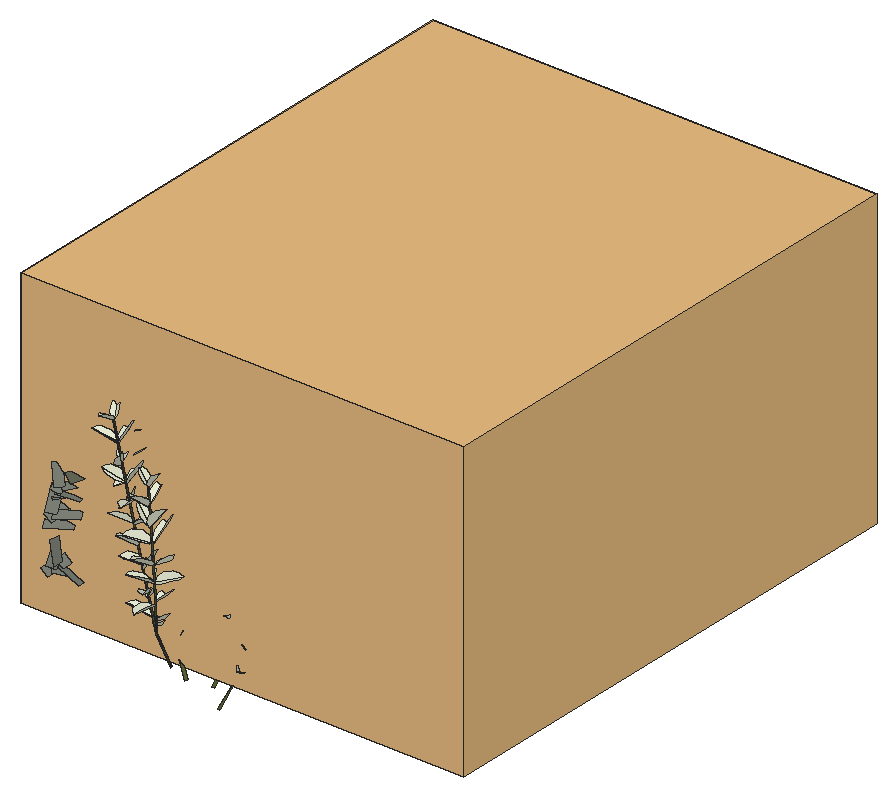
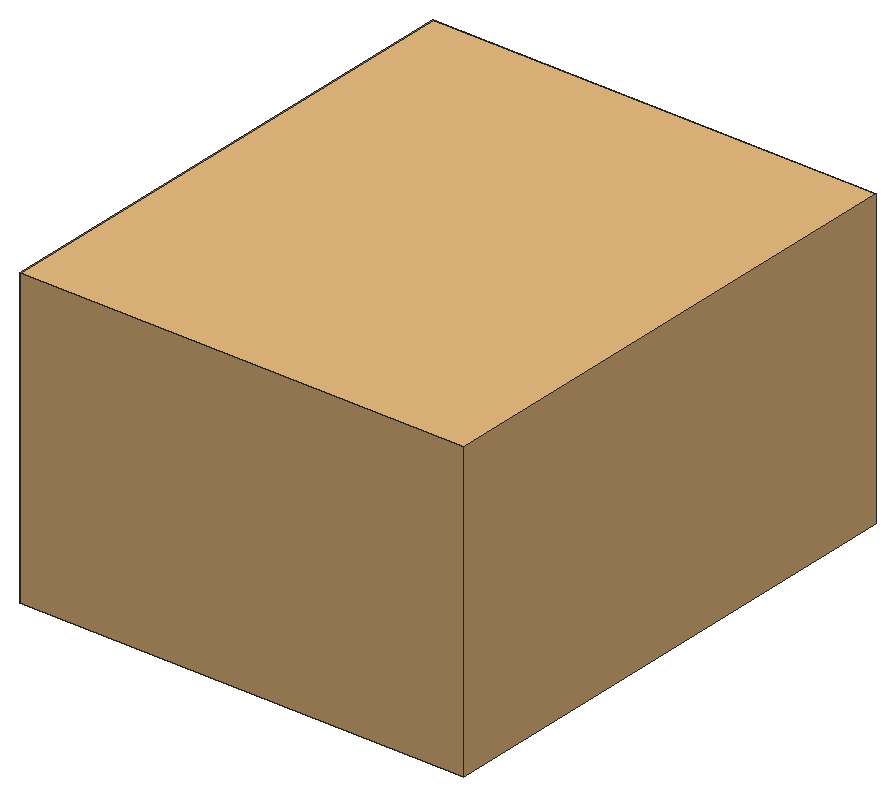
# SketchUp Ruby script. Lengths in inches.
U = 1.inch
M = Sketchup.active_model
def pt(a) = Geom::Point3d.new(a.map { |v| v * U })
def face(e, loops, mat)
  f = e.add_face(loops[0].map { |a| pt(a) })
  loops[1..].each { |l| e.add_face(l.map { |a| pt(a) }).erase! }
  f.material = f.back_material = mat if mat
  f
end
# faces: each face lists its corners as indices into pts; further lists are holes
def faces(e, pts, list, mat = nil) = list.each { |f| face(e, (f[0].is_a?(Array) ? f : [f]).map { |l| l.map { |i| pts[i] } }, mat) }
# xy, xz, yz: faces in a plane at the given z, y or x. An outline is a flat list of corners, or four numbers for a rectangle; further outlines are holes
def ring(l) = l.size == 4 ? [[l[0], l[1]], [l[2], l[1]], [l[2], l[3]], [l[0], l[3]]] : l.each_slice(2).to_a
def flat(e, list, mat, &to3) = list.each { |f| face(e, (f[0].is_a?(Array) ? f : [f]).map { |l| ring(l).map { |u, v| to3.(u, v) } }, mat) }
def xy(e, z, list, mat = nil) = flat(e, list, mat) { |x, y| [x, y, z] }
def xz(e, y, list, mat = nil) = flat(e, list, mat) { |x, z| [x, y, z] }
def yz(e, x, list, mat = nil) = flat(e, list, mat) { |y, z| [x, y, z] }
def lines(e, pts, list) = list.each { |a, b| e.add_line(pt(pts[a]), pt(pts[b])) }
# prism: a flat outline (further loops are holes) pulled along v
def prism(e, loops, v, mat = nil)
  f = face(e, loops, mat); d = Geom::Vector3d.new(v.map { |x| x * U })
  f.pushpull(f.normal.samedirection?(d) ? d.length : -d.length)
end
def box(e, o, s, mat = nil) = prism(e, [[o, [o[0] + s[0], o[1], o[2]], [o[0] + s[0], o[1] + s[1], o[2]], [o[0], o[1] + s[1], o[2]]]], [0, 0, s[2]], mat)
def at(x, y, z, deg = 0) = Geom::Transformation.translation(pt([x, y, z])) * Geom::Transformation.rotation(ORIGIN, Z_AXIS, deg.degrees)
def axes(o, x, y, z) = Geom::Transformation.new([*x, 0, *y, 0, *z, 0, *pt(o).to_a, 1])
def part(name) = M.definitions.add(name)
# library, detail: a bought-in or finely detailed component or shape, given as its bounding box
def library(name, o, s) = part(name).tap { |d| box(d.entities, o, s) }
def detail(e, o, s) = box(e.add_group.entities, o, s)
def put(e, d, t, mat = nil) = e.add_instance(d, t).tap { |i| i.material = mat if mat }
def group(e, t, mat = nil) = e.add_group.tap { |g| g.transformation = t; g.material = mat if mat }.entities
root = M.entities
M.materials.add("0ad16as01f6asdLeafVar1sfd015as60f1as6").color = [231, 235, 211]
M.materials.add("asdfasdf0165f6asdLeafVar1sfd015as60f1as6").color = [231, 235, 211]
M.materials.add("dw_stemssadfasdfa0sdf1s01d6w1").color = [90, 97, 50]
M.materials.add("viburnumblaasdfas0df1w06d").color = [98, 102, 84]
M.materials.add("viburnumbladsadfasdfad0w122").color = [125, 129, 119]
c1 = part("vdw_leaf\#3")
p = [[0,0,0],[-2.77,1.61,2.32],[-4.3125,6.1,4.5],[-3.97,13.49,6.09],[-2.47,18.57,6.3],[-0.2,22.73,5.75],
  [2.54,19.66,6.85],[4.3,15.93,7.09],[5.03,7.6,5.43],[3.32,1.76,2.74]]
faces(c1.entities,p,[[0,1,2,3,4,5],[0,5,6,7,8,9]],"asdfasdf0165f6asdLeafVar1sfd015as60f1as6")
c2 = part("dw_brancj_2\#2")
p = [[9.7,-0.22,29.95],[0.23,-1.96,0.34],[-0.05,1.51,0.11],[9.65,1.51,29.46],[18.64,-8.75,84.43],[18.96,-6.63,84.625],
  [1.53,6.02,63.68],[1.42,8.18,63.25],[-10.58,8.77,161.17],[-10.41,9.98,160.68],[26.34,-9.37,211.72],[26.57,-8.28,211.23]]
faces(c2.entities,p,[[0,1,2],[0,2,3],[4,0,3],[4,3,5],[6,0,3],[6,3,7],[8,6,7],[8,7,9],
  [10,4,5],[10,5,11]],"dw_stemssadfasdfa0sdf1s01d6w1")
c3 = part("vdw_branch2\#3")
put(c3.entities,c1,axes([19.53,-5.9,102.42],[1.12377,-0.50004,0],[0.46097,1.03596,0.47664],[-0.19377,-0.43548,1.13389]))
put(c3.entities,c1,axes([-5.89,6.52,109.44],[-1.07209,0.83679,0],[-0.77141,-0.98832,0.52702],[0.32427,0.41545,1.25373]))
put(c3.entities,c1,axes([-0.44,8.23,75.28],[0.88709,-0.9947,0],[0.92159,0.82189,0.33087],[-0.25219,-0.22491,1.26111]))
put(c3.entities,c1,axes([24.71,-8.97,190.81],[-0.82641,0.91101,0],[-0.83983,-0.76184,0.47664],[0.35303,0.32025,1.13389]))
put(c3.entities,c1,axes([-2.29,8.24,91.35],[1.24603,-0.47303,0],[0.43826,1.15445,0.33087],[-0.11993,-0.31592,1.26111]))
put(c3.entities,c1,axes([12.26,-3.11,37.92],[-0.64625,1.02205,0.22511],[-1.04383,-0.61044,-0.22511],[-0.07533,-0.30931,1.18809]))
put(c3.entities,c1,axes([26.17,-9.17,210.27],[-0.99452,-0.10453,0],[0.09636,-0.91681,0.38752],[-0.04051,0.38539,0.92186]))
put(c3.entities,c1,axes([-6.07,9.4,125.35],[-0.90214,-0.98107,0],[0.90896,-0.83583,0.33087],[-0.24874,0.22873,1.26111]))
put(c3.entities,c1,axes([-4.13,7.29,110.58],[0.44715,-1.078,0.64369],[1.05816,0.63649,0.33087],[-0.58725,0.40856,1.09216]))
put(c3.entities,c1,axes([23.91,-8.22,171.96],[0.62307,0.85009,-0.63406],[-0.71531,0.8798,0.47664],[0.78296,0.12729,0.94004]))
put(c3.entities,c2,at(-0.09,0.18,-0.25),"dw_stemssadfasdfa0sdf1s01d6w1")
put(c3.entities,c1,axes([23.34,-9.65,156.59],[-0.31364,-1.00782,0.58216],[1.10369,-0.17062,0.29925],[-0.17137,0.6239,0.98776]))
put(c3.entities,c1,axes([15.03,-3.37,58.83],[-1.05425,-0.00194,0.58442],[-0.14303,-1.11707,-0.26172],[0.55355,-0.3046,0.99755]))
put(c3.entities,c1,axes([-11.625,9.46,160.37],[0.36812,0.92978,0],[-0.85713,0.33936,0.38752],[0.3603,-0.14265,0.92186]))
put(c3.entities,c1,axes([21.32,-8.53,138.72],[1.21379,0.19904,0],[-0.19904,1.21379,0],[0,0,1.23]))
put(c3.entities,c1,axes([22.54,-9.2,141.43],[-1.02887,0.17955,0.60182],[-0.23387,-1.13057,-0.06253],[0.56696,-0.17376,1.02111]))
put(c3.entities,c1,axes([23.9,-8.82,173.84],[-1.14567,-0.37474,0],[0.35918,-1.0981,0.04438],[-0.01409,0.04308,1.17993]))
put(c3.entities,c1,axes([-7.84,8.92,143.59],[-1.26971,0.40522,0],[-0.37543,-1.17638,0.33087],[0.10274,0.32192,1.26111]))
put(c3.entities,c1,axes([19.77,-8.01,85.98],[-0.32405,-1.14591,0.18674],[1.10278,-0.32969,-0.10948],[0.15845,0.14442,1.16117]))
put(c3.entities,c1,axes([-0.62,5.76,76.34],[-0.08879,1.17576,-0.67771],[-1.34525,-0.16582,-0.11144],[-0.17897,0.66309,1.17383]))
put(c3.entities,c1,axes([20.49,-8.22,121.07],[0.39924,-0.78471,-0.8233],[1.08735,0.33121,0.2116],[0.09035,-0.83005,0.83495]))
put(c3.entities,c1,axes([15.15,-3.72,62.9],[1.16251,0.40128,-0.0211],[-0.39924,1.16074,0.07874],[0.0456,-0.06757,1.2273]))
put(c3.entities,c1,axes([20.72,-8.08,120.26],[-0.03693,1.2277,-0.06551],[-1.22944,-0.03698,0],[-0.00197,0.06548,1.22825]))
put(c3.entities,c1,axes([22.58,-8.36,155.57],[-0.56247,1.09386,0],[-1.00839,-0.51852,0.47664],[0.42389,0.21796,1.13389]))
put(c3.entities,c1,axes([3.97,3.13,57.96],[-1.09459,0.76041,0],[-0.72262,-1.0402,-0.1735],[-0.10109,-0.14552,1.29352]))
put(c3.entities,c1,axes([-10.8,9.06,160.75],[-0.66334,-0.72138,0],[0.66835,-0.61458,0.24329],[-0.1829,0.16818,0.92729]))
put(c3.entities,c1,axes([19.06,-9.3125,103.96],[-1.01345,0.25553,-0.60051],[-0.2265,-1.12952,-0.09839],[-0.59598,0.03076,1.01889]))
put(c3.entities,c1,axes([18.07,-6.2,81.7],[-0.56247,1.09386,0],[-1.00839,-0.51852,0.47664],[0.42389,0.21796,1.13389]))
put(c3.entities,c1,axes([12.95,-0.39,43.31],[0.13044,-1.19832,0],[1.11025,0.12085,0.29925],[-0.30382,-0.03307,1.14057]))
put(c3.entities,c1,axes([2.28,8.28,56.18],[1.32413,-0.31027,0],[0.30923,1.31968,-0.11144],[0.02542,0.1085,1.35543]))
put(c3.entities,c1,axes([-7.55,9.96,143.07],[1.34251,-0.21744,0],[0.20045,1.23761,0.52702],[-0.08426,-0.52024,1.25373]))
put(c3.entities,c1,axes([26.15,-8.25,210.66],[0.94661,-0.25364,0],[0.235,0.87703,0.24329],[-0.06431,-0.24,0.92729]))
put(c3.entities,c1,axes([-6.48,11.37,125.16],[0.64635,1.10315,0.46356],[-1.16569,0.46153,0.52702],[0.27017,-0.6478,1.16488]))
put(c3.entities,c1,axes([25.74,-8.35,191.28],[0.13044,-1.19832,0],[1.11025,0.12085,0.29925],[-0.30382,-0.03307,1.14057]))
put(c3.entities,c1,axes([-5.125,7.47,91.6],[-1.10024,0.63688,0.48318],[-0.78682,-1.00808,-0.46292],[0.14137,-0.65404,1.184]))
c4 = part("Component\#315")
p = [[0.25,0,0],[2.05,0.01,0.35],[1.81,4.2,1.66],[0,4.19,1.3125]]
faces(c4.entities,p,[[0,1,2,3]],"viburnumbladsadfasdfad0w122")
c5 = part("viburnumblad2")
put(c5.entities,c4,axes([-19.23,-4.49,-32.18],[83.35428,0,0],[0,79.38502,0],[0,0,83.35428]))
c6 = part("Component\#314")
p = [[0.14,0,0],[2.58,0.05,0.25],[2.44,5.11,2.64],[0,5.05,2.39]]
faces(c6.entities,p,[[0,1,2,3]],"viburnumblaasdfas0df1w06d")
c7 = part("viburnumblad1\#2")
put(c7.entities,c6,axes([-37.25,6.23,19.31],[75.98784,0,0],[0,65.50676,0],[0,0,75.98784]))
c8 = part("vdw_leaf\#1")
p = [[0,0,0],[-2.77,1.61,2.32],[-4.3125,6.1,4.5],[-3.97,13.49,6.09],[-2.47,18.57,6.3],[-0.2,22.73,5.75],
  [2.54,19.66,6.85],[4.3,15.93,7.09],[5.03,7.6,5.43],[3.32,1.76,2.74]]
faces(c8.entities,p,[[0,1,2,3,4,5],[0,5,6,7,8,9]],"0ad16as01f6asdLeafVar1sfd015as60f1as6")
c9 = part("dw_branch_3\#2")
p = [[-10.06,-1.6,62.9],[-0.2,1.54,-0.01],[-10.43,1.54,62.72],[0.18,-1.6,0.17],[-23.75,-21.66,88.91],[-25.7,-20.3,89.55],
  [13.4,11.62,104.56],[13.33,13.52,104.47],[-49.25,-41.87,130.3125],[-50.33,-40.21,130.71],[-4.97,21.13,143.98],[35.61,27.99,178.64],
  [-5.09,23.64,143.96],[35.32,29.14,178.46],[-67.7,-55.38,181.06],[-68.34,-54.45,181.62],[-22.8125,33.9,200.59],[-22.94,35.79,200.41],
  [56.61,36.78,229.75],[56.29,38.09,229.57],[-70.63,-67.46,248.85],[-70.72,-66.33,249.5],[-25.05,43.32,240.75],[-24.98,44.26,240.57]]
faces(c9.entities,p,[[0,1,2],[0,3,1],[4,2,5],[4,0,2],[6,0,2],[6,2,7],[8,4,5],[8,5,9],
  [10,6,7],[11,6,7],[10,7,12],[11,7,13],[14,8,9],[14,9,15],[16,10,12],[16,12,17],
  [18,11,13],[18,13,19],[20,14,15],[20,15,21],[22,16,17],[22,17,23]],"dw_stemssadfasdfa0sdf1s01d6w1")
c10 = part("dw_branch3\#2")
put(c10.entities,c8,axes([-70.33,-63.58,233.32],[-1.00752,0.412,0.78596],[-0.24851,-1.22189,0.32195],[0.83141,0.09817,1.01433]))
put(c10.entities,c8,axes([-66.93,-54.91,182.82],[-0.84976,-0.98359,0.33619],[0.99572,-0.74889,0.32577],[-0.05223,0.46521,1.22907]))
put(c10.entities,c8,axes([-46.12,-39.49,126.35],[1.23843,0.5364,0.23552],[-0.56438,0.94474,0.81599],[0.15707,-0.83465,1.07498]))
put(c10.entities,c8,axes([13.0625,13.13,104.77],[-1.01271,0.69982,-0.26884],[-0.74268,-0.99813,0.19939],[-0.10222,0.31872,1.21473]))
put(c10.entities,c8,axes([-18.87,30.42,186.42],[0.36309,1.06515,-0.56675],[-1.14134,0.49515,0.19939],[0.39128,0.45593,1.10754]))
put(c10.entities,c8,axes([-3.2,4.15,75.77],[-1.04153,0.55414,0.44243],[-0.23365,-1.01045,0.71554],[0.6695,0.50943,0.93801]))
put(c10.entities,c8,axes([23.2,19.41,136.3],[-0.65687,-1.11295,-0.05714],[1.05857,-0.61429,-0.20411],[0.15163,-0.1536,1.24868]))
put(c10.entities,c8,axes([-25.57,35.48,201.32],[-0.64726,0.62827,0.87973],[-0.71635,-1.0172,0.19939],[0.80962,-0.39773,0.87973]))
put(c10.entities,c8,axes([-36.37,-32.14,110.35],[-0.80747,1.09962,0.12544],[-0.83333,-0.50188,-0.96467],[-0.72833,-0.64487,0.96467]))
put(c10.entities,c8,axes([-9.89,26.72,156.79],[0.45529,1.02969,0.56572],[-1.16919,0.33753,0.32662],[0.11537,-0.64297,1.07744]))
put(c10.entities,c8,axes([-26.57,46.1,241.0625],[0.00015,0.80921,0.22536],[-0.83985,0.00446,-0.01542],[-0.01605,-0.22532,0.80906]))
put(c10.entities,c8,axes([-9.2,-2.58,61.06],[-1.10001,-0.40312,0.39014],[0.40883,-1.1116,0.00411],[0.35732,0.13566,1.14763]))
put(c10.entities,c8,axes([-69.91,-63.11,233.93],[1.36249,-0.1432,0],[0.13201,1.25603,0.5309],[-0.05549,-0.52799,1.26295]))
put(c10.entities,c8,axes([32.2,25.46,166.13],[0.06878,-1.29051,-0.05714],[1.22165,0.07415,-0.20411],[0.2113,-0.04403,1.24868]))
put(c10.entities,c8,axes([-5.68,-0.66,44.43],[-0.48448,-1.12287,0.17078],[0.98138,-0.33653,0.57135],[-0.48308,0.36756,1.04626]))
put(c10.entities,c8,axes([43.45,32.81,198.64],[0.5408,1.19584,0.14106],[-0.94242,0.32409,0.86557],[0.74952,-0.45533,0.98656]))
put(c10.entities,c8,axes([12.52,14.14,104.98],[1.02694,0.54888,0.41092],[-0.53566,1.05407,-0.06927],[-0.38969,-0.12321,1.13846]))
put(c10.entities,c8,axes([44.55,32.375,198.73],[-0.65687,-1.11295,-0.05714],[1.05857,-0.61429,-0.20411],[0.15163,-0.1536,1.24868]))
put(c10.entities,c8,axes([-5.67,21.17,141.44],[-1.10726,0.43603,-0.32953],[-0.49537,-1.03435,0.29588],[-0.17521,0.40597,1.12589]))
put(c10.entities,c8,axes([55.69,37.84,229.48],[0.18984,0.96334,0.18958],[-0.71996,0.0053,0.69399],[0.66755,-0.26823,0.69457]))
put(c10.entities,c8,axes([-21.52,36.85,205.2],[0.72606,-0.98817,0.14519],[0.94364,0.7084,0.10251],[-0.16885,0.05176,1.19664]))
put(c10.entities,c8,axes([-68.51,-56.35,196.07],[1.16319,0.72381,0],[-0.66725,1.0723,0.5309],[0.28049,-0.45075,1.26295]))
put(c10.entities,c9,at(0.01,-0.09,-0.02),"dw_stemssadfasdfa0sdf1s01d6w1")
put(c10.entities,c8,axes([-2.49,5.18,75.91],[0.78614,-0.90346,-0.30078],[0.86953,0.79562,-0.11715],[0.28546,-0.14014,1.16705]))
put(c10.entities,c8,axes([-23.125,-16.22,82.25],[0.32175,1.32576,0.12544],[-1.33153,0.31835,0.05068],[0.01989,-0.13382,1.3633]))
put(c10.entities,c8,axes([-23.75,41.99,230.3],[0.85958,-0.87451,0.14519],[0.66531,0.75721,0.62192],[-0.54076,-0.36226,1.01955]))
put(c10.entities,c8,axes([27.07,22.48,149.34],[0.92952,-0.64745,-0.62467],[0.50188,1.074,-0.36637],[0.71693,0.02135,1.04468]))
put(c10.entities,c8,axes([17.66,16.25,119.93],[-0.91649,0.83891,-0.3601],[-0.87434,-0.77966,0.40896],[0.0492,0.54447,1.14321]))
put(c10.entities,c8,axes([-68.37,-54.54,181.63],[0.32047,1.28399,0.35434],[-1.33153,0.31835,0.05068],[-0.03484,-0.35624,1.32241]))
put(c10.entities,c8,axes([-28.98,-27.1,96.48],[-0.8814,-0.35966,-0.98523],[0.75246,-1.11336,-0.26672],[-0.73065,-0.71272,0.91382]))
put(c10.entities,c8,axes([-15.23,28.43,172.72],[-1.21149,0.11898,0.32517],[-0.09739,-1.25259,0.09551],[0.33228,0.0667,1.21356]))
put(c10.entities,c8,axes([-17.5625,31.23,186.85],[-0.49275,-1.12287,0.14519],[0.95014,-0.33653,0.62192],[-0.53717,0.36756,1.01955]))
put(c10.entities,c8,axes([26.7,21.22,149.39],[-1.00104,0.22334,0.83093],[0.36894,-1.0402,0.72406],[0.77731,0.78134,0.72643]))
put(c10.entities,c8,axes([-31.125,-24.87,97.38],[0.75482,-0.86936,0.69068],[-0.00159,0.80023,1.00899],[-1.08766,-0.58016,0.45842]))
put(c10.entities,c8,axes([-71.21,-66.73,248.67],[0.25207,0.96771,0],[-0.8921,0.23237,0.38752],[0.375,-0.09768,0.92186]))
put(c10.entities,c8,axes([-24.11,41.05,229.55],[-1.11612,0.51924,-0.26884],[-0.56394,-1.10897,0.19939],[-0.15444,0.29694,1.21473]))
put(c10.entities,c8,axes([6.75,8.37,91.63],[-0.33418,-1.12287,0.39014],[1.13558,-0.33653,0.00411],[0.10478,0.36756,1.14763]))
put(c10.entities,c8,axes([-26,45.89,241.63],[-0.26986,-0.70824,-0.32129],[0.56818,-0.39091,0.38449],[-0.49365,-0.09775,0.63011]))
put(c10.entities,c8,axes([3.74,17.32,124.35],[0.22441,1.22913,-0.16274],[-1.07812,0.11178,-0.64246],[-0.61228,0.25367,1.07162]))
put(c10.entities,c8,axes([-5.44,22.27,140.88],[1.2203,0.00475,0.31374],[-0.097,1.20386,0.35905],[-0.29841,-0.37189,1.1663]))
put(c10.entities,c8,axes([-13.79,29.35,173.31],[0.83169,-0.90108,0.14519],[0.68877,0.73594,0.62192],[-0.55187,-0.34509,1.01955]))
put(c10.entities,c8,axes([-16.92,-7.26,72.98],[1.30647,0.30378,-0.27886],[0.07026,0.74892,1.14503],[0.40633,-1.10623,0.69861]))
put(c10.entities,c8,axes([4.8,17.55,125.22],[-0.25598,-1.17842,0.26559],[1.01553,-0.08455,0.60363],[-0.56975,0.35087,1.00767]))
put(c10.entities,c8,axes([5.3125,8.35,91.45],[0.00638,1.22913,-0.27714],[-1.16413,0.11178,0.46895],[0.48205,0.25367,1.13617]))
put(c10.entities,c8,axes([38.12,30.57,183.07],[1.12534,0.26182,-0.63833],[-0.46674,1.18829,-0.33545],[0.5081,0.51169,1.10563]))
put(c10.entities,c8,axes([-70.41,-60.38,214.47],[-0.41425,1.30587,0],[-1.20383,-0.38188,0.5309],[0.50605,0.16053,1.26295]))
put(c10.entities,c8,axes([37.03,28.75,180.67],[-1.12533,0.00102,-0.63799],[-0.00113,-1.2408,0],[-0.62497,0.00057,1.10237]))
put(c10.entities,c8,axes([30.71,25.35,165.96],[-0.1364,1.29314,0.22715],[-1.08768,-0.23921,0.70862],[0.73536,-0.11394,1.09026]))
put(c10.entities,c8,axes([-38.05,-30.84,110.67],[-0.31533,-1.27379,-0.2839],[1.018,-0.40311,0.67794],[-0.74394,-0.05723,1.08307]))
put(c10.entities,c8,axes([50.11,34.45,213.36],[-1.05669,0.74401,-0.05714],[-0.616,-0.82138,0.69675],[0.37221,0.60904,1.04705]))
put(c10.entities,c8,axes([-65.32,-58.78,200.07],[-1.14597,-0.19668,-0.6713],[0.21784,-1.26924,0],[-0.64812,-0.11124,1.139]))
put(c10.entities,c8,axes([-53.2,-43.37,143.59],[-0.72817,-1.09167,-0.2839],[0.82127,-0.72411,0.67794],[-0.71934,0.19815,1.08307]))
put(c10.entities,c8,axes([-61.1,-50.25,163.67],[-0.52887,1.19686,-0.30066],[-1.10762,-0.57104,-0.32484],[-0.42634,0.12264,1.23812]))
put(c10.entities,c8,axes([-54.12,-42.96,142.67],[0.32175,1.32576,0.12544],[-1.33153,0.31835,0.05068],[0.01989,-0.13382,1.3633]))
put(c10.entities,c8,axes([22.03,20.08,132.3],[1.17066,0.5058,-0.34078],[-0.35758,1.16671,0.50333],[0.49407,-0.35407,1.17172]))
put(c10.entities,c8,axes([-8.59,26.04,158.21],[-0.49275,-1.12287,0.14519],[0.95014,-0.33653,0.62192],[-0.53717,0.36756,1.01955]))
put(c10.entities,c8,axes([49.92,34.03,213.7],[1.24742,-0.35176,0.25024],[0.42127,1.159,-0.4708],[-0.09426,0.52477,1.20753]))
put(c10.entities,c8,axes([-70.34,-67.02,249.05],[-0.57048,-0.79684,0],[0.73827,-0.52855,0.24329],[-0.20203,0.14464,0.92729]))
put(c10.entities,c8,axes([56.04,36.81,228.63],[0.33451,-0.90845,-0.15237],[0.87636,0.33365,-0.06538],[0.11487,-0.11636,0.94597]))
put(c10.entities,c8,axes([-69.93,-60.58,214.88],[-0.45293,-0.99272,-0.78227],[1.14635,-0.58199,0.07483],[-0.40282,-0.65636,1.06615]))
put(c10.entities,c8,axes([-16.77,-8.59,72.7],[-1.22785,0.11509,0.53076],[-0.24879,-1.22495,-0.30991],[0.46742,-0.38989,1.16587]))
put(c10.entities,c8,axes([18.29,17.18,119.24],[1.19981,-0.45946,0.3029],[0.40159,1.22775,0.27158],[-0.37626,-0.1547,1.25575]))
put(c10.entities,c8,axes([-6.73,-0.68,43.74],[0.05346,1.22913,-0.27201],[-1.22696,0.11178,0.26396],[0.28163,0.25367,1.20164]))
put(c10.entities,c8,axes([-58.57,-48.42,160.98],[0.43385,-1.23789,0.39533],[1.04879,0.57965,0.66404],[-0.76727,0.09236,1.13122]))
put(c10.entities,c8,axes([-23.4,38.49,215.38],[0.06762,1.22913,-0.26884],[-1.23909,0.11178,0.19939],[0.21835,0.25367,1.21473]))
put(c10.entities,c8,axes([-22.21,-16.62,83.17],[-0.72817,-1.09167,-0.2839],[0.82127,-0.72411,0.67794],[-0.71934,0.19815,1.08307]))
put(c10.entities,c8,axes([-45.7,-40.77,126.53],[-1.33715,-0.0713,-0.0976],[0.07167,-1.28508,-0.04314],[-0.09306,-0.0492,1.31098]))
put(c10.entities,c8,axes([-22.39,38.51,216.12],[-0.49275,-1.12287,0.14519],[0.95014,-0.33653,0.62192],[-0.53717,0.36756,1.01955]))
c11 = part("vdw_leaf\#2")
p = [[0,0,0],[-2.77,1.61,2.32],[-4.3125,6.1,4.5],[-3.97,13.49,6.09],[-2.47,18.57,6.3],[-0.2,22.73,5.75],
  [2.54,19.66,6.85],[4.3,15.93,7.09],[5.03,7.6,5.43],[3.32,1.76,2.74]]
faces(c11.entities,p,[[0,1,2,3,4,5],[0,5,6,7,8,9]],"asdfasdf0165f6asdLeafVar1sfd015as60f1as6")
c12 = part("dg_branch_1\#2")
p = [[46.12,1.57,35.62],[46,5.42,35.41],[0.14,1.79,0.05],[0.26,-2.0625,0.27],[74.05,2.99,75.8],[74.11,5.28,75.58],
  [103.46,0.47,94.74],[104.03,2.92,94.84],[81.14,16.92,120.46],[81.2,18.78,120.24],[130.47,-5.6875,130.27],[130.58,-3.66,129.85],
  [80.82,34.4375,191.22],[80.64,35.93,190.9],[148.49,-14.56,203.24],[148.9,-12.8125,203.11],[81.08,37.95,226.93],[81.4,39.1,227.03],
  [157.45,-18.19,250.77],[157.7,-17.01,250.41]]
faces(c12.entities,p,[[0,1,2,3],[4,0,1],[4,1,5],[6,4,5],[6,5,7],[8,4,5],[8,5,9],[10,6,7],
  [10,7,11],[12,8,9],[12,9,13],[14,10,11],[14,11,15],[16,12,13],[16,13,17],[18,14,15],
  [18,15,19]],"dw_stemssadfasdfa0sdf1s01d6w1")
c13 = part("vdw_branch1\#3")
put(c13.entities,c11,axes([120.69,-2.42,117.31],[1.12221,-0.24063,-0.65809],[0.19207,1.24776,-0.12871],[0.65778,0.01392,1.11658]))
put(c13.entities,c11,axes([81,38.9,226.05],[0.7888,-0.58155,0],[0.48308,0.65523,0.47],[-0.28484,-0.38635,0.83138]))
put(c13.entities,c11,axes([78.08,12.69,106.05],[-1.43826,-0.02353,-0.03177],[0.0088,-1.31777,0.57755],[-0.03854,0.57714,1.31741]))
put(c13.entities,c11,axes([130.18,-4.73,130.41],[-0.38031,-1.29044,-0.11242],[1.20662,-0.31032,-0.51987],[0.47109,-0.24694,1.24081]))
put(c13.entities,c11,axes([157.08,-17.89,249.93],[-0.91355,0.40674,0],[-0.37496,-0.84216,0.38752],[0.15762,0.35401,0.92186]))
put(c13.entities,c11,axes([90.64,3.03,86.49],[0.32514,-0.85045,-0.99675],[0.69523,0.98247,-0.61148],[1.11061,-0.36604,0.67459]))
put(c13.entities,c11,axes([80.15,28.42,160.95],[-0.16039,0.95636,-1.06292],[-1.41646,0.03966,0.24943],[0.19509,1.07422,0.93709]))
put(c13.entities,c11,axes([126.74,-5.45,129.22],[-0.59819,0.96152,-0.6841],[-0.85772,0.12575,0.92675],[0.75427,0.88089,0.57856]))
put(c13.entities,c11,axes([133.22,-6.12,150.66],[-0.93823,0.76985,0.59124],[-0.47726,-1.08188,0.65135],[0.84525,0.24366,1.02405]))
put(c13.entities,c11,axes([80.43,22.89,141.32],[-1.42571,-0.19312,0.01373],[0.18338,-1.31425,0.5561],[-0.0621,0.5528,1.32692]))
put(c13.entities,c11,axes([33.14,0.88,26.42],[-0.13338,1.31536,0.04876],[-1.04528,-0.13221,0.7073],[0.72315,0.03348,1.07497]))
put(c13.entities,c11,axes([152.63,-15.08,221.76],[-1.28188,0.41945,0.0579],[-0.3638,-1.18547,0.53367],[0.21665,0.49113,1.23869]))
put(c13.entities,c11,axes([80.05,28.28,160.33],[-0.46732,-1.26661,0.40679],[1.27397,-0.40257,0.21004],[-0.07408,0.44645,1.30501]))
put(c13.entities,c11,axes([153.95,-14.8,235.875],[0.39005,1.07743,0.20605],[-0.96443,0.25296,0.50293],[0.42961,-0.3464,0.99807]))
put(c13.entities,c11,axes([80.2,24.22,141.74],[1.33062,-0.46576,0.02628],[0.44746,1.2746,-0.06608],[-0.00197,0.0722,1.37936]))
put(c13.entities,c11,axes([145.48,-12.5,188.92],[-1.32952,0.16983,0.16138],[-0.09299,-1.2361,0.53471],[0.21503,0.51548,1.22904]))
put(c13.entities,c11,axes([139.64,-9.18,171.24],[0.05682,1.30088,0.23414],[-1.13176,-0.05343,0.57151],[0.58357,-0.22963,1.13417]))
put(c13.entities,c11,axes([70.95,4.35,71.98],[-1.1081,-0.41873,0.64752],[0.33675,-1.28259,-0.25313],[0.6937,-0.04625,1.15721]))
put(c13.entities,c11,axes([59.85,4.55,56.17],[-0.26797,1.24526,0.35754],[-0.9369,-0.41634,0.74783],[0.83377,-0.10389,0.98674]))
put(c13.entities,c11,axes([33.11,3.36,25.66],[-0.57817,-1.07968,-0.5679],[1.11554,-0.21356,-0.7297],[0.49375,-0.78178,0.98363]))
put(c13.entities,c12,at(-0.21,0.34,-0.17),"dw_stemssadfasdfa0sdf1s01d6w1")
put(c13.entities,c11,axes([80.91,19.01,122.53],[-0.84258,1.13222,-0.27981],[-1.15093,-0.75138,0.42537],[0.18861,0.47293,1.3457]))
put(c13.entities,c11,axes([119.8,-1.22,114.1],[-1.3235,-0.25012,0.09101],[0.25933,-1.31572,0.15537],[0.05991,0.1698,1.33794]))
put(c13.entities,c11,axes([46.29,5.1,38.04],[0.98937,0.73827,-0.47585],[-0.72359,1.03721,0.10473],[0.44068,0.18581,1.20453]))
put(c13.entities,c11,axes([81.1875,33.03,184.45],[1.33883,0.26986,0.35053],[-0.09581,1.22087,-0.57399],[-0.42216,0.53228,1.20262]))
put(c13.entities,c11,axes([80.16,36.28,206.98],[-0.83993,0.85737,-0.6234],[-1.05964,-0.65701,0.5241],[0.02941,0.81391,1.07976]))
put(c13.entities,c11,axes([154.86,-16.15,234.87],[0.02509,-1.15302,-0.28506],[1.1487,-0.04894,0.29908],[-0.30202,-0.28195,1.11384]))
put(c13.entities,c11,axes([108.77,-0.33,101.14],[-0.47691,-1.03266,-0.72709],[1.25395,-0.29455,-0.40416],[0.15052,-0.81814,1.06325]))
put(c13.entities,c11,axes([89.79,3.01,85.87],[-0.61344,0.75518,0.8965],[-0.17758,-1.01824,0.73622],[1.13385,0.22574,0.58569]))
put(c13.entities,c11,axes([81.56,20.31,123.29],[0.37259,-1.3435,0.21057],[1.29385,0.32364,-0.22445],[0.16906,0.25791,1.34638]))
put(c13.entities,c11,axes([46.45,1.82,36.74],[-0.77883,0.29892,1.0614],[0.19124,-1.24314,0.49044],[1.08598,0.43329,0.67484]))
put(c13.entities,c11,axes([71.37,4.02,72.32],[0.72905,0.81546,-0.74421],[-0.66805,0.98958,0.42988],[0.8391,0.14186,0.97745]))
put(c13.entities,c11,axes([136.59,-5.88,150.53],[0.85845,-0.99897,-0.12437],[0.96526,0.81273,0.13453],[-0.02572,-0.18182,1.28292]))
put(c13.entities,c11,axes([80.375,38.8,225.86],[-0.25178,0.96778,0],[-0.89216,-0.23211,0.38752],[0.37503,0.09757,0.92186]))
put(c13.entities,c11,axes([74.43,7.99,85.38],[-1.05703,0.91669,-0.33543],[-0.95806,-0.87958,0.61531],[0.18697,0.6754,1.25659]))
put(c13.entities,c11,axes([76.57,9.74,89.32],[0.63146,-1.21538,0.33508],[1.18148,0.49387,-0.43517],[0.26321,0.48577,1.26593]))
put(c13.entities,c11,axes([81.6875,36.97,207.4],[0.09422,-1.04424,0.38486],[1.01646,0.1939,0.27727],[-0.33299,0.33382,0.98727]))
put(c13.entities,c11,axes([157.29,-17.17,249.98],[0.50586,-0.50586,0],[0.38853,0.38853,0.41105],[-0.29684,-0.29684,0.56115]))
put(c13.entities,c11,axes([79.92,15.8,106.09],[1.03917,-0.29343,-0.90675],[-0.14587,1.22131,-0.5624],[0.92163,0.5191,0.88824]))
put(c13.entities,c11,axes([61.95,3.88,56.26],[0.41243,-1.28546,0],[1.17466,0.37688,-0.54831],[0.5221,0.16751,1.23363]))
put(c13.entities,c11,axes([151.99,-14.79,208.15],[-0.48571,-1.21723,-0.32393],[1.25386,-0.50033,0],[-0.12005,-0.30087,1.31056]))
put(c13.entities,c11,axes([108.44,0.62,102.22],[0.82183,0.96078,0.38967],[-0.62327,0.08618,1.10203],[0.79141,-0.88661,0.51693]))
put(c13.entities,c11,axes([145.6,-10.56,188.62],[1.03241,-0.02554,-0.82693],[0.3944,1.11584,0.45794],[0.70325,-0.61672,0.89706]))
put(c13.entities,c11,axes([78.59,32.3,183.89],[-1.12675,-0.42036,0.43987],[0.5899,-0.98149,0.57312],[0.14901,0.70693,1.05726]))
put(c13.entities,c11,axes([152.08,-13.42,223.37],[0.79993,-0.44251,-0.69938],[0.68456,0.82615,0.26026],[0.41048,-0.60953,0.85515]))
put(c13.entities,c11,axes([140.71,-8.74,170.55],[0.41903,-1.24177,-0.32393],[1.26224,0.33728,0.33986],[-0.23168,-0.40836,1.26573]))
put(c13.entities,c11,axes([149.25,-12.53,205.78],[1.24456,0.38285,0.23414],[-0.42999,1.04826,0.57151],[-0.02056,-0.62679,1.13417]))
c14 = library("Broadleaf plant",[0,0,0],[62.33,72.62,41.59])
put(root,c3,axes([1264.7,211.69,1.63],[-0.15667,-0.0351,-0.03733],[0.03572,-0.15945,0],[-0.0296,-0.00663,0.19757]))
put(root,c5,axes([1243.54,209.6,13.17],[-0.00141,0.01241,-0.00136],[-0.00618,0.00049,0.01093],[0.01085,0.0019,0.00605]))
put(root,c5,axes([1241.98,208.93,22.71],[0.00909,0.00791,-0.00471],[-0.00403,0.00937,0.00796],[0.00828,-0.00412,0.00905]))
put(root,c5,axes([1242.55,210.46,22.72],[0.00501,-0.0098,-0.00679],[0.00996,0.00749,-0.00346],[0.00656,-0.00389,0.01045]))
put(root,c5,axes([1243.51,211.78,12.62],[0.00141,-0.01241,0.00136],[0.00862,-0.00002,-0.00914],[0.00903,0.00196,0.00851]))
put(root,c5,axes([1240.52,210.82,20.19],[0.00481,-0.00941,-0.00652],[0.01076,0.00809,-0.00374],[0.00656,-0.00389,0.01045]))
put(root,c5,axes([1242.61,211.82,25.53],[0.00283,-0.01146,-0.00038],[0.01049,0.00275,-0.00491],[0.00467,0.00082,0.00968]))
put(root,c5,axes([1241.04,210,21.625],[0.00997,-0.00134,-0.00814],[0.0038,0.01207,0.00267],[0.00731,-0.00445,0.00969]))
put(root,c5,axes([1243,210.01,27.11],[0.00489,0.00995,-0.00397],[-0.0081,0.00635,0.00558],[0.00694,0.00038,0.0084]))
put(root,c5,axes([1241.88,209.74,12.66],[0.00427,0.00859,-0.00811],[-0.005,0.00913,0.00703],[0.0107,0.00084,0.00653]))
put(root,c5,axes([1241.77,211.13,12.4],[0.00627,-0.00896,-0.00619],[0.00573,0.0092,-0.00751],[0.00942,0.00088,0.00827]))
put(root,c5,axes([1241.9,210.41,26.07],[0.00974,0.00261,-0.006],[-0.00192,0.01057,0.00135],[0.0062,-0.00026,0.0089]))
put(root,c5,axes([1240.53,210.13,11.74],[0.00716,-0.00025,-0.0097],[-0.0002,0.01356,-0.00049],[0.01011,0.00042,0.00745]))
put(root,c5,axes([1241.34,211.22,24.93],[0.00761,-0.00572,-0.00506],[0.00557,0.01001,-0.00285],[0.00619,-0.00075,0.00889]))
put(root,c5,axes([1242.85,211.49,27.03],[0.00889,-0.00626,-0.00451],[0.00557,0.01001,-0.00285],[0.00526,-0.00007,0.00943]))
put(root,c5,axes([1242.85,210.9,13.76],[0.00745,-0.00026,-0.01011],[-0.00018,0.01255,-0.00046],[0.01011,0.00042,0.00745]))
put(root,c7,axes([1243.68,211.52,28.38],[0.01127,-0.00662,-0.00498],[0.00702,0.01432,-0.0031],[0.00548,-0.00011,0.01154]))
put(root,c5,axes([1241.43,216.08,18.53],[-0.0065,0.00265,0.00695],[0.00166,-0.0098,0.00501],[0.00741,0.00415,0.00458]))
put(root,c5,axes([1243.47,216.5625,19.75],[-0.00677,0.00276,0.00724],[0.00154,-0.00908,0.00464],[0.00741,0.00415,0.00458]))
put(root,c5,axes([1242.29,216.95,18.99],[-0.00435,-0.00477,0.00798],[0.00611,-0.00825,-0.00162],[0.00685,0.00405,0.00535]))
put(root,c5,axes([1242.28,215.9,19.51],[-0.00523,0.00868,0.00226],[-0.00357,-0.00459,0.00897],[0.00802,0.00357,0.00411]))
put(root,c10,axes([1270.75,215.58,3.91],[0.09481,-0.08589,0.04174],[0.08433,0.10034,0.02262],[-0.03765,0.00844,0.15579]))
put(root,c5,axes([1242.92,217.75,19.86],[0.00062,-0.00952,0.00405],[0.00764,-0.00238,-0.00656],[0.00666,0.00333,0.00596]))
put(root,c5,axes([1242.82,216.16,20.79],[-0.00062,0.00952,-0.00405],[-0.0058,0.00311,0.00781],[0.00831,0.00266,0.0042]))
put(root,c13,axes([1267.875,211.61,0.51],[-0.11174,0.0797,0],[-0.0797,-0.11174,0],[0,0,0.16889]))
put(root,c5,axes([1241.42,217.48,19.83],[0.00523,-0.00868,-0.00226],[0.00529,0.00516,-0.00737],[0.00696,0.00241,0.00605]))
put(root,c5,axes([1241.48,216.13,20.39],[0.00435,0.00477,-0.00798],[-0.00392,0.00825,0.00263],[0.00812,0.00193,0.0048]))
put(root,c5,axes([1242.26,217.34,20.9],[0.00677,-0.00276,-0.00724],[0.0003,0.00981,-0.00339],[0.00756,0.00183,0.00557]))
put(root,c3,axes([1275.69,209.81,-1.1],[0.02729,0.1244,-0.09048],[-0.14364,0.03151,0],[0.01575,0.07182,0.15671]))
put(root,c5,axes([1243.14,222.21,28.26],[-0.00855,-0.00095,0.00486],[0.00394,-0.00929,0.00471],[0.00385,0.00566,0.0068]))
put(root,c5,axes([1241.72,222.125,29.15],[0.00769,0.00057,-0.00539],[-0.00261,0.00972,-0.00258],[0.00555,0.0035,0.00706]))
put(root,c3,axes([1271.59,213.63,-0.375],[0.0097,0.14118,-0.10053],[-0.16302,0.01121,0],[0.0056,0.08151,0.17413]))
put(root,c5,axes([1242.27,223.29,29.58],[0.00853,-0.00582,-0.00111],[0.00461,0.00781,-0.00517],[0.00374,0.00366,0.00797]))
put(root,c14,axes([1234.07,212.62,1.89],[1.41,0,0],[0,1.41,0],[0,0,1.41]))
put(root,c5,axes([1244.52,270.73,30.06],[-0.00372,-0.00756,-0.00527],[0.01001,-0.00205,-0.00401],[0.00166,-0.0069,0.00731]))
put(root,c5,axes([1242.51,274.89,23.72],[-0.00968,0.00131,0.00494],[-0.00285,-0.01022,-0.00281],[0.00419,-0.00363,0.00837]))
put(root,c7,axes([1242.58,275.27,25.6875],[-0.00299,-0.01191,-0.00429],[0.01424,-0.00187,-0.0047],[0.00288,-0.00486,0.01046]))
put(root,c7,axes([1241.98,273.44,27.34],[0.00886,-0.00621,-0.00526],[0.00932,0.00889,0.00498],[0.00073,-0.00681,0.00878]))
put(root,c5,axes([1242.19,276.3,23.07],[-0.0092,-0.00594,0.0008],[0.00497,-0.0084,-0.00522],[0.00323,-0.00386,0.00866]))
put(root,c5,axes([1242.15,275.98,24.48],[-0.00334,-0.0097,-0.00381],[0.01007,-0.00189,-0.00393],[0.0026,-0.00465,0.00851]))
put(root,c5,axes([1241.59,277.62,28.69],[-0.01126,-0.00309,0.00036],[0.00297,-0.01108,-0.00222],[0.00093,-0.00205,0.01147]))
put(root,c5,axes([1240.09,275.8125,12.3],[0.00083,-0.00664,-0.00958],[0.01085,0.00394,-0.00179],[0.00425,-0.00877,0.00644]))
put(root,c5,axes([1241.22,277.23,22.63],[-0.00331,-0.00841,-0.00433],[0.01007,-0.00189,-0.00393],[0.00222,-0.00567,0.00805]))
put(root,c13,axes([1259.64,288.83,0.51],[0.01907,-0.13922,0],[0.13922,0.01907,0],[0,0,0.17291]))
put(root,c5,axes([1240.8125,276.5,23.74],[0.00449,-0.00779,-0.00619],[0.00881,0.00487,0.00016],[0.00266,-0.00553,0.00801]))
put(root,c5,axes([1240.91,275.41,24.71],[0.00968,-0.00131,-0.00494],[0.00378,0.00904,0.00475],[0.00337,-0.00599,0.00744]))
put(root,c7,axes([1243.625,278.79,27.5],[-0.00543,0.00233,0.01137],[0.00034,-0.01453,0.00314],[0.0116,0.00141,0.00526]))
put(root,c5,axes([1240.07,278.18,25.98],[-0.00385,-0.0119,-0.00772],[0.01402,-0.00199,-0.00394],[0.00214,-0.0084,0.01187]))
put(root,c5,axes([1240.92,278.75,27.55],[-0.00596,-0.00978,-0.00229],[0.01005,-0.00579,-0.00143],[0.00006,-0.0027,0.01137]))
put(root,c5,axes([1240.14,276.74,22.73],[0.01011,-0.00136,-0.00516],[0.0034,0.00814,0.00428],[0.00337,-0.00599,0.00744]))
put(root,c7,axes([1244.95,279.95,29.11],[-0.00364,-0.00823,0.00913],[0.00776,-0.0108,-0.00665],[0.01031,0.00314,0.00694]))
put(root,c7,axes([1238.92,280.97,17.79],[-0.00228,-0.0125,-0.00287],[0.01428,-0.00152,-0.00471],[0.00336,-0.00314,0.01093]))
